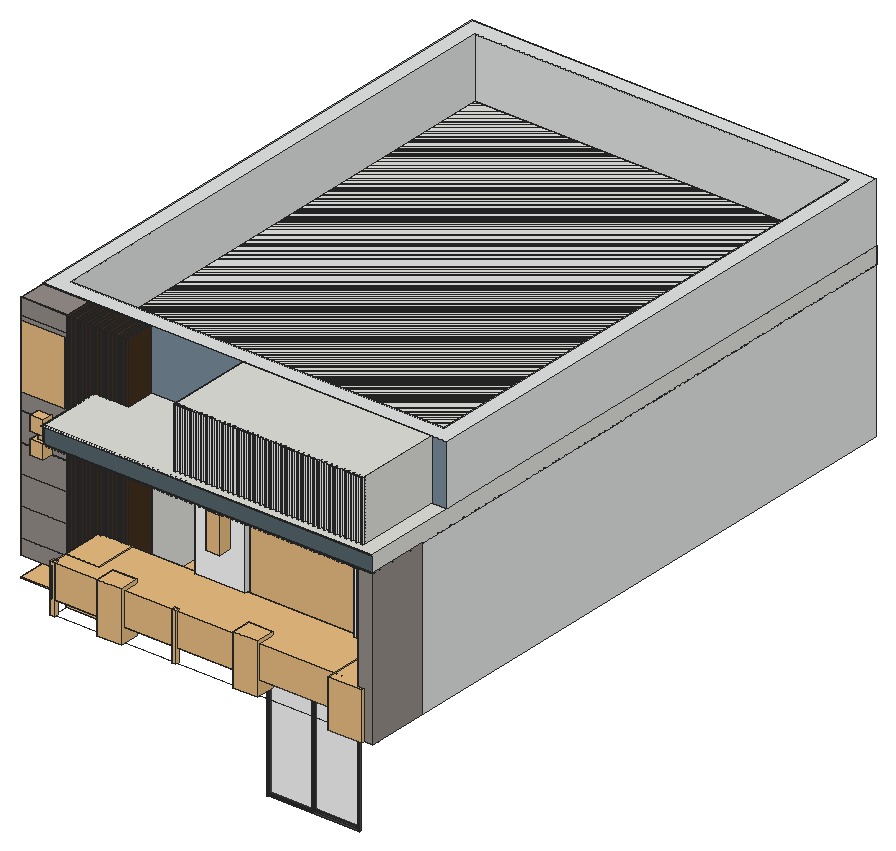
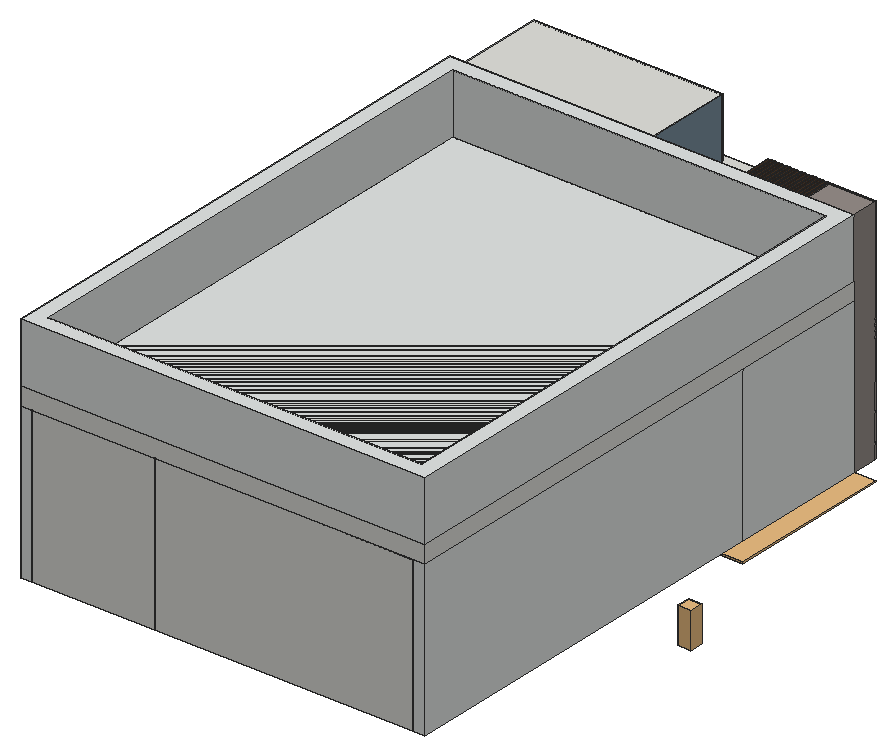
# SketchUp Ruby script. Lengths in inches.
U = 1.inch
M = Sketchup.active_model
def pt(a) = Geom::Point3d.new(a.map { |v| v * U })
def face(e, loops, mat)
  f = e.add_face(loops[0].map { |a| pt(a) })
  loops[1..].each { |l| e.add_face(l.map { |a| pt(a) }).erase! }
  f.material = f.back_material = mat if mat
  f
end
# faces: each face lists its corners as indices into pts; further lists are holes
def faces(e, pts, list, mat = nil) = list.each { |f| face(e, (f[0].is_a?(Array) ? f : [f]).map { |l| l.map { |i| pts[i] } }, mat) }
# xy, xz, yz: faces in a plane at the given z, y or x. An outline is a flat list of corners, or four numbers for a rectangle; further outlines are holes
def ring(l) = l.size == 4 ? [[l[0], l[1]], [l[2], l[1]], [l[2], l[3]], [l[0], l[3]]] : l.each_slice(2).to_a
def flat(e, list, mat, &to3) = list.each { |f| face(e, (f[0].is_a?(Array) ? f : [f]).map { |l| ring(l).map { |u, v| to3.(u, v) } }, mat) }
def xy(e, z, list, mat = nil) = flat(e, list, mat) { |x, y| [x, y, z] }
def xz(e, y, list, mat = nil) = flat(e, list, mat) { |x, z| [x, y, z] }
def yz(e, x, list, mat = nil) = flat(e, list, mat) { |y, z| [x, y, z] }
def lines(e, pts, list) = list.each { |a, b| e.add_line(pt(pts[a]), pt(pts[b])) }
# prism: a flat outline (further loops are holes) pulled along v
def prism(e, loops, v, mat = nil)
  f = face(e, loops, mat); d = Geom::Vector3d.new(v.map { |x| x * U })
  f.pushpull(f.normal.samedirection?(d) ? d.length : -d.length)
end
def box(e, o, s, mat = nil) = prism(e, [[o, [o[0] + s[0], o[1], o[2]], [o[0] + s[0], o[1] + s[1], o[2]], [o[0], o[1] + s[1], o[2]]]], [0, 0, s[2]], mat)
def at(x, y, z, deg = 0) = Geom::Transformation.translation(pt([x, y, z])) * Geom::Transformation.rotation(ORIGIN, Z_AXIS, deg.degrees)
def axes(o, x, y, z) = Geom::Transformation.new([*x, 0, *y, 0, *z, 0, *pt(o).to_a, 1])
def part(name) = M.definitions.add(name)
# library, detail: a bought-in or finely detailed component or shape, given as its bounding box
def library(name, o, s) = part(name).tap { |d| box(d.entities, o, s) }
def detail(e, o, s) = box(e.add_group.entities, o, s)
def put(e, d, t, mat = nil) = e.add_instance(d, t).tap { |i| i.material = mat if mat }
def group(e, t, mat = nil) = e.add_group.tap { |g| g.transformation = t; g.material = mat if mat }.entities
root = M.entities
M.materials.add("Kamosho - kamn7918 33.43cm").color = [255, 255, 255]
M.materials.add("Marble C 150cm").color = [150, 142, 138]
M.materials.add("Plain White Flat 3698829 28cm").color = [227, 230, 229]
M.materials.add("Wall Paint Bumpy 01 Blue 100cm").color = [86, 103, 109]
M.materials.add("Wall Paint Dusk Blue Satin 300cm").color = [122, 143, 157]
M.materials.add("Wood 011 26.84cm").color = [255, 255, 255]
M.materials.add("Wood Amboyan 13.2cm").color = [255, 255, 255]
M.materials.add("Wood Tiles Dark Shiny 03 100cm").color = [68, 48, 33]
M.materials.add("[0135_DarkGray]").color = [81, 81, 81]
M.materials.add("[Translucent Glass Gray]").color = [128, 128, 128]
M.materials["[Translucent Glass Gray]"].alpha = 0.1
c1 = part("PENTEK_RP Fineline 50S_Sliding_DoorCase_E1")
box(c1.entities,[0,0,0],[1.51,3.66,99.27],"[0135_DarkGray]")
c2 = part("PENTEK_RP Fineline 50S_SlidingDooe_Case_E2")
box(c2.entities,[0,0,0],[96.25,3.66,1.51],"[0135_DarkGray]")
c3 = part("pentek_RP Fineline 50S_SlidingDoor_Case")
put(c3.entities,c1,at(97.76,0,0))
put(c3.entities,c2,at(1.51,0,0))
put(c3.entities,c1,at(0,0,0))
put(c3.entities,c2,at(1.51,0,97.76))
c4 = part("PENTEK_RP Fineline 50S_SlidingDoor_GlazingBead_2")
box(c4.entities,[0,0,0],[0.56,0.59,94.39],"[0135_DarkGray]")
c5 = part("PENTEK_RP Fineline 50S_SlidingDoor_Glass")
box(c5.entities,[0,0,0],[46.58,0.16,94.39],"[Translucent Glass Gray]")
c6 = part("PENTEK_RP Fineline 50S_SlidingDoor_GlazingBead")
box(c6.entities,[0,0,0],[45.47,0.59,0.56],"[0135_DarkGray]")
c7 = part("PENTEK_RP Fineline 50S_SlidingDoor_Leaf_E1")
xy(c7.entities,0,[[0,0,0.93,1.97],[0.93,1.57,1.49,1.97]],"[0135_DarkGray]")
xy(c7.entities,96.25,[[0,0,0.93,0,0.93,1.57,1.49,1.57,1.49,1.97,0,1.97]],"[0135_DarkGray]")
xz(c7.entities,0,[[0,0,0.93,96.25]],"[0135_DarkGray]")
xz(c7.entities,1.57,[[0.93,0,1.49,95.32],[0.93,95.32,1.49,96.25]],"[0135_DarkGray]")
xz(c7.entities,1.97,[[0,0,1.49,96.25]],"[0135_DarkGray]")
yz(c7.entities,0,[[0,0,1.97,96.25]],"[0135_DarkGray]")
yz(c7.entities,0.93,[[0,0,1.57,0.93],[0,0.93,1.57,95.32],[0,95.32,1.57,96.25]],"[0135_DarkGray]")
yz(c7.entities,1.49,[[1.57,0,1.97,95.32],[1.57,95.32,1.97,96.25]],"[0135_DarkGray]")
c8 = part("PENTEK_RP Fineline 50S_SlidingDoor_Leaf_E2")
xy(c8.entities,0,[[0,0,0,1.57,0.56,1.57,0.56,1.97,46.02,1.97,46.02,1.57,46.58,1.57,46.58,0]],"[0135_DarkGray]")
xy(c8.entities,0.93,[[0,0,46.58,1.57]],"[0135_DarkGray]")
xy(c8.entities,1.49,[[0.56,1.57,46.02,1.97]],"[0135_DarkGray]")
xz(c8.entities,0,[[0,0,46.58,0.93]],"[0135_DarkGray]")
xz(c8.entities,1.57,[[0,0,0.56,0.93],[46.02,0,46.58,0.93],[0.56,0.93,46.02,1.49]],"[0135_DarkGray]")
xz(c8.entities,1.97,[[0.56,0,46.02,1.49]],"[0135_DarkGray]")
yz(c8.entities,0,[[0,0,1.57,0.93]],"[0135_DarkGray]")
yz(c8.entities,0.56,[[1.57,0,1.97,0.93],[1.57,0.93,1.97,1.49]],"[0135_DarkGray]")
yz(c8.entities,46.02,[[1.57,0,1.97,0.93],[1.57,0.93,1.97,1.49]],"[0135_DarkGray]")
yz(c8.entities,46.58,[[0,0,1.57,0.93]],"[0135_DarkGray]")
c9 = part("PENTEK_RP Fineline S_SlidingDoor_Leaf1")
put(c9.entities,c4,at(0.93,0,0.93))
put(c9.entities,c4,at(46.96,0,0.93))
put(c9.entities,c5,at(1.49,1.42,0.93))
put(c9.entities,c6,at(1.49,0,0.93))
put(c9.entities,c5,at(1.49,0.59,0.93))
put(c9.entities,c7,at(0,0,0))
put(c9.entities,c7,axes([48.44,0,0],[-1,0,0],[0,1,0],[0,0,1]))
put(c9.entities,c8,axes([0.93,0,96.25],[1,0,0],[0,1,0],[0,0,-1]))
put(c9.entities,c8,at(0.93,0,0))
put(c9.entities,c6,at(1.49,0,94.77))
c10 = part("PENTEK_RP Fineline 50S_SlidingDoor_Leaf2")
put(c10.entities,c5,at(1.49,1.42,0.93))
put(c10.entities,c6,at(1.49,0,94.77))
put(c10.entities,c4,at(46.96,0,0.93))
put(c10.entities,c5,at(1.49,0.59,0.93))
put(c10.entities,c4,at(0.93,0,0.93))
put(c10.entities,c7,at(0,0,0))
put(c10.entities,c7,axes([48.44,0,0],[-1,0,0],[0,1,0],[0,0,1]))
put(c10.entities,c6,at(1.49,0,0.93))
put(c10.entities,c8,axes([0.93,0,96.25],[1,0,0],[0,1,0],[0,0,-1]))
put(c10.entities,c8,at(0.93,0,0))
c11 = library("Group\#41",[0,0,0],[10.21,10.21,27.95])
c12 = library("Tlon Light 1950 Ceiling 152 010",[-38.39,-38.39,-3.78],[76.78,76.78,3.41])
c13 = library("Group\#39",[0,0,0],[138,129.875,1])
c14 = library("Potted Plant 13",[-10,-7.28,0],[18.93,15.17,39.22])
c15 = library("Door 243 065",[-19.36,-2.49,0],[38.72,4.98,81.96])
c16 = library("Potted Plant 08",[-13.67,-16.93,0],[26.14,33.37,37.04])
c17 = part("Group\#8")
box(c17.entities,[0,0,0],[96,4.5,120])
c18 = part("Group\#4")
box(c18.entities,[0,0,0],[201,9,120])
c19 = part("Group\#7")
prism(c19.entities,[[[6,4.5,0],[0,4.5,0],[0,4.5,120],[96,4.5,120],[96,4.5,0],[36,4.5,0],[36,4.5,84],[6,4.5,84]]],[0,-4.5,0])
c20 = part("Group\#9")
box(c20.entities,[0,0,0],[96,4.5,120])
c21 = part("Group\#6")
xy(c21.entities,0,[[0,0,90,4.5],[126,0,126,4.5,132,4.5,132,148.5,136.5,148.5,136.5,64.5,160.5,64.5,160.5,60,136.5,60,136.5,0],[190.5,60,190.5,64.5,196.5,64.5,196.5,148.5,201,148.5,201,60]])
xy(c21.entities,84,[[90,0,126,4.5],[160.5,60,190.5,64.5]])
xy(c21.entities,120,[[0,0,136.5,0,136.5,60,201,60,201,148.5,196.5,148.5,196.5,64.5,136.5,64.5,136.5,148.5,132,148.5,132,4.5,0,4.5]])
xz(c21.entities,0,[[0,0,90,0,90,84,126,84,126,0,136.5,0,136.5,120,0,120]])
xz(c21.entities,4.5,[[0,0,0,120,132,120,132,0,126,0,126,84,90,84,90,0]])
xz(c21.entities,60,[[136.5,0,160.5,0,160.5,84,190.5,84,190.5,0,201,0,201,120,136.5,120]])
xz(c21.entities,64.5,[[136.5,0,136.5,120,196.5,120,196.5,0,190.5,0,190.5,84,160.5,84,160.5,0]])
xz(c21.entities,148.5,[[132,0,136.5,120],[196.5,0,201,120]])
yz(c21.entities,0,[[0,0,4.5,120]])
yz(c21.entities,90,[[0,0,4.5,84]])
yz(c21.entities,126,[[0,0,4.5,84]])
yz(c21.entities,132,[[4.5,0,148.5,120]])
yz(c21.entities,136.5,[[0,0,60,120],[64.5,0,148.5,120]])
yz(c21.entities,160.5,[[60,0,64.5,84]])
yz(c21.entities,190.5,[[60,0,64.5,84]])
yz(c21.entities,196.5,[[64.5,0,148.5,120]])
yz(c21.entities,201,[[60,0,148.5,120]])
c22 = part("Vertical panel")
xy(c22.entities,0,[[0,-14.875,2.125,7]])
xy(c22.entities,180,[[0,-14.875,2.125,7]],"Wood Tiles Dark Shiny 03 100cm")
xz(c22.entities,-14.875,[[0,0,2.125,180]],"Wood Tiles Dark Shiny 03 100cm")
xz(c22.entities,7,[[0,0,2.125,180]])
yz(c22.entities,0,[[-14.875,0,7,180]],"Wood Tiles Dark Shiny 03 100cm")
yz(c22.entities,2.125,[[-14.875,0,7,180]],"Wood Tiles Dark Shiny 03 100cm")
c23 = library("Ploe",[1045.01,-6.26,132],[3.15,3.15,37.57])
c24 = part("Group74\#1")
put(c24.entities,c23,at(0,0,0))
put(c24.entities,c23,at(-82.72,0,0))
put(c24.entities,c23,at(-145.86,0,0))
put(c24.entities,c23,at(-240.58,0,0))
put(c24.entities,c23,at(-240.58,45.25,0))
c25 = library("Group75\#1",[805.22,-5.47,143.61],[241.37,46.03,25.18])
c26 = library("DOOR 1",[0,0,0],[82.68,3.9375,84.65])
c27 = library("Spot Light",[-5.1,-5.1,-11.05],[10.2,10.2,11.05])
c28 = library("Lamp Wall Outdoor 94-02",[-1.89,-4.65,-3.17],[3.78,4.65,6.35])
c29 = library("Group\#46",[0,0,0],[39.25,57.0625,1])
c30 = part("Railing baluster")
box(c30.entities,[0,-1,0],[1.1875,1,46.5625],"Wood 011 26.84cm")
xz(root,519.27,[[726.46,251,726.46,252,778.5,252,778.5,251.71,778.26,251.71,778.26,251,776.76,251,776.76,251.71,774.66,251.71,774.66,251,773.16,251,773.16,251.71,771.07,251.71,771.07,251,769.57,251,769.57,251.71,767.48,251.71,767.48,251,765.98,251,765.98,251.78,763.89,251.78,763.89,251,762.39,251,762.39,251.78,760.3,251.78,760.3,251,758.8,251,758.8,251.78,756.7,251.78,756.7,251,755.2,251,755.2,251.78,753.11,251.78,753.11,251,751.61,251,751.61,251.78,749.52,251.78,749.52,251,748.02,251,748.02,251.84,745.93,251.84,745.93,251,744.43,251,744.43,251.84,742.33,251.84,742.33,251,740.83,251,740.83,251.84,738.74,251.84,738.74,251,737.24,251,737.24,251.9,735.15,251.9,735.15,251,733.65,251,733.65,251.9,731.56,251.9,731.56,251,730.06,251,730.06,251.9,727.96,251.9,727.96,251]])
p = [[702.93,344.15,132],[702.93,389.4,132],[766.07,344.15,132],[829.21,344.15,132],[892.36,344.15,132],[955.5,344.15,132],
  [937,374.15,251],[937,354.02,251],[675.04,389.4,296.28],[675.04,389.4,246.07]]
lines(root,p,[[0,1],[0,2],[2,3],[3,4],[4,5],[6,7],[8,9]])
g1 = group(root,at(831,391.58,30))
put(g1,c3,axes([0,0.19,0],[0.72528,0,0],[0,0.49,0],[0,0,0.87512]))
put(g1,c9,axes([1.09,0,1.32],[0.72528,0,0],[0,0.49,0],[0,0,0.87512]))
put(g1,c10,axes([35.77,0.96,1.32],[0.72528,0,0],[0,0.49,0],[0,0,0.87512]))
put(root,c11,at(679.38,511.15,42.52))
put(root,c12,axes([680.94,422.85,115.7],[0.1475,0,0],[0,0.1475,0],[0,0,0.1475]))
put(root,c12,axes([680.94,477.57,115.7],[0.1475,0,0],[0,0.1475,0],[0,0,0.1475]))
put(root,c12,axes([756.5,477.34,115.75],[0.1475,0,0],[0,0.1475,0],[0,0,0.1475]))
put(root,c12,axes([753.27,421.48,115.93],[0.1475,0,0],[0,0.1475,0],[0,0,0.1475]))
put(root,c13,at(640.5,389.4,115.875),"Wood Amboyan 13.2cm")
put(root,c14,at(854.5,349.05,132))
put(root,c14,at(749.45,347.88,132))
put(root,c15,axes([754.52,524.28,132],[0.92977,0,0],[0,-0.44,0],[0,0,1.02]))
put(root,c16,at(715.56,373.65,132))
put(root,c16,at(936.14,353.56,132))
g2 = group(root,at(640.5,339.27,132))
put(g2,c17,at(210,486,0))
put(g2,c18,at(9,481.5,0))
g3 = group(g2,at(306,0,0))
box(g3,[0,48,0],[9,442.5,120],"Plain White Flat 3698829 28cm")
put(g2,c19,at(210,433.5,0))
g4 = group(g2,at(0,0,0))
box(g4,[0,180,0],[9,310.5,120],"Plain White Flat 3698829 28cm")
put(g2,c20,at(210,225,0))
g5 = group(g2,at(9,48,0))
xy(g5,0,[[129,0,129,132,123,132,123,141,138,141,138,9,297,9,297,0],[0,132,87,141]])
xy(g5,6,[[167.625,0,253.5,9]])
xy(g5,84,[[87,132,123,141]])
xy(g5,112.4375,[[167.625,0,253.5,9]])
xy(g5,120,[[129,0,297,0,297,9,138,9,138,141,0,141,0,132,129,132]])
xz(g5,0,[[[129,0,297,120],[167.625,6,253.5,112.4375]]],"Kamosho - kamn7918 33.43cm")
xz(g5,9,[[[138,0,297,120],[167.625,6,253.5,112.4375]]])
xz(g5,132,[[0,0,87,0,87,84,123,84,123,0,129,0,129,120,0,120]],"Kamosho - kamn7918 33.43cm")
xz(g5,141,[[0,0,0,120,138,120,138,0,123,0,123,84,87,84,87,0]])
yz(g5,0,[[132,0,141,120]])
yz(g5,87,[[132,0,141,84]])
yz(g5,123,[[132,0,141,84]])
yz(g5,129,[[0,0,132,120]],"Kamosho - kamn7918 33.43cm")
yz(g5,138,[[9,0,141,120]])
yz(g5,167.625,[[0,6,9,112.4375]])
yz(g5,253.5,[[0,6,9,112.4375]])
yz(g5,297,[[0,0,9,120]])
put(g2,c21,at(9,333,0))
g6 = group(root,at(640.5,404.27,132))
box(g6,[0,-13.875,0],[35.9375,20.875,180],"Marble C 150cm")
g7 = group(root,at(640.5,389.4,132),"Marble C 150cm")
box(g7,[34.54,0,123.52],[1.4,1,21.92],"Marble C 150cm")
xy(g7,0,[[0,0,35.9375,1]],"Marble C 150cm")
xy(g7,12,[[0,0,35.9375,1]],"Marble C 150cm")
xy(g7,12.31,[[0,0,35.9375,1]],"Marble C 150cm")
xy(g7,34.24,[[0,0,35.9375,1]],"Marble C 150cm")
xy(g7,34.56,[[0,0,35.9375,1]],"Marble C 150cm")
xy(g7,56.48,[[0,0,35.9375,1]],"Marble C 150cm")
xy(g7,56.8,[[0,0,35.9375,1]],"Marble C 150cm")
xy(g7,78.72,[[0,0,35.9375,1]],"Marble C 150cm")
xy(g7,79.04,[[0,0,35.9375,1]],"Marble C 150cm")
xy(g7,100.96,[[0,0,35.9375,1]],"Marble C 150cm")
xy(g7,101.28,[[0,0,35.9375,1]],"Marble C 150cm")
xy(g7,114.07,[[0,0,34.54,1]],"Marble C 150cm")
xy(g7,123.2,[[34.54,0,35.9375,1]],"Marble C 150cm")
xy(g7,145.76,[[34.54,0,35.9375,1]],"Marble C 150cm")
xy(g7,164.28,[[0,0,34.54,1]],"Marble C 150cm")
xy(g7,167.69,[[0,0,35.9375,1]],"Marble C 150cm")
xy(g7,168,[[0,0,35.9375,1]],"Marble C 150cm")
xy(g7,180,[[0,0,35.9375,1]],"Marble C 150cm")
xz(g7,0,[[0,0,35.9375,12],[0,12.31,35.9375,34.24],[0,34.56,35.9375,56.48],[0,56.8,35.9375,78.72],[0,79.04,35.9375,100.96],
  [0,101.28,35.9375,101.28,35.9375,123.2,34.54,123.2,34.54,114.07,0,114.07],[34.54,145.76,35.9375,145.76,35.9375,167.69,0,167.69,0,164.28,34.54,164.28],[0,168,35.9375,180]],"Marble C 150cm")
xz(g7,1,[[0,0,35.9375,12],[0,12,35.9375,12.31],[0,12.31,35.9375,34.24],[0,34.24,35.9375,34.56],[0,34.56,35.9375,56.48],
  [0,56.48,35.9375,56.8],[0,56.8,35.9375,78.72],[0,78.72,35.9375,79.04],[0,79.04,35.9375,100.96],[0,100.96,35.9375,101.28],
  [0,101.28,0,114.07,34.54,114.07,34.54,123.2,35.9375,123.2,35.9375,101.28],[34.54,145.76,34.54,164.28,0,164.28,0,167.69,35.9375,167.69,35.9375,145.76],[0,167.69,35.9375,168],[0,168,35.9375,180]],"Marble C 150cm")
yz(g7,0,[[0,0,1,12],[0,12.31,1,34.24],[0,34.56,1,56.48],[0,56.8,1,78.72],[0,79.04,1,100.96],
  [0,101.28,1,114.07],[0,164.28,1,167.69],[0,168,1,180]],"Marble C 150cm")
yz(g7,34.54,[[0,114.07,1,123.2],[0,145.76,1,164.28]],"Marble C 150cm")
yz(g7,35.9375,[[0,0,1,12],[0,12.31,1,34.24],[0,34.56,1,56.48],[0,56.8,1,78.72],[0,79.04,1,100.96],
  [0,101.28,1,123.2],[0,145.76,1,167.69],[0,168,1,180]],"Marble C 150cm")
p = [[35.9375,1,123.52],[35.9375,1,123.2],[35.9375,1,145.76],[35.9375,1,145.44],[34.54,0,123.52],[34.54,0,123.2],
  [34.54,0,145.76],[34.54,0,145.44]]
lines(g7,p,[[0,1],[2,3],[4,5],[6,7]])
g8 = group(root,at(676.44,389.4,132))
put(g8,c22,at(46.49,14.875,0))
put(g8,c22,at(34.69,14.875,0))
put(g8,c22,at(31.8,14.875,0))
put(g8,c22,at(37.58,14.875,0))
put(g8,c22,at(43.36,14.875,0))
put(g8,c22,at(0,14.875,0),"Wood Tiles Dark Shiny 03 100cm")
put(g8,c22,at(23.13,14.875,0))
put(g8,c22,at(20.24,14.875,0))
put(g8,c22,at(40.47,14.875,0))
put(g8,c22,at(17.35,14.875,0))
put(g8,c22,at(28.91,14.875,0))
put(g8,c22,at(26.02,14.875,0))
put(g8,c22,at(8.67,14.875,0))
put(g8,c22,at(2.89,14.875,0),"Wood Tiles Dark Shiny 03 100cm")
put(g8,c22,at(5.78,14.875,0))
put(g8,c22,at(11.5625,14.875,0))
put(g8,c22,at(14.45,14.875,0))
g9 = group(root,at(943.5,339.27,132),"Marble C 150cm")
prism(g9,[[[0,0,0],[12,0,0],[12,0,120],[0,0,120],[0,0,119]]],[0,48,0])
g10 = group(root,at(640.5,411.27,132))
xy(g10,120,[[0,0,85.93,0,85.93,108,81.43,108,81.43,9,9,9,9,108,0,108]])
xz(g10,0,[[0,0,85.93,120]])
xz(g10,9,[[9,0,81.43,120]])
xz(g10,108,[[0,0,9,120],[81.43,0,85.93,120]])
yz(g10,0,[[0,0,108,120]],"Plain White Flat 3698829 28cm")
yz(g10,9,[[9,0,108,120]])
yz(g10,81.43,[[9,0,108,120]])
yz(g10,85.93,[[0,0,108,120]])
g11 = group(root,at(701.35,342.57,132))
put(g11,c24,at(-804.4375,6.26,-132))
put(g11,c25,at(-804.4375,6.26,-132))
g12 = group(root,at(903,386.27,132),"Wood 011 26.84cm")
prism(g12,[[[0,1,0],[40.5,1,0],[40.5,0,0],[38.5,0,0],[38.5,0.5,0],[36.65,0.5,0],[36.65,0,0],[34.65,0,0],[34.65,0.5,0],[32.8,0.5,0],[32.8,0,0],[30.8,0,0],[30.8,0.5,0],[28.95,0.5,0],[28.95,0,0],[26.95,0,0],[26.95,0.5,0],[25.1,0.5,0],[25.1,0,0],[23.1,0,0],[23.1,0.5,0],[21.25,0.5,0],[21.25,0,0],[19.25,0,0],[19.25,0.5,0],[17.4,0.5,0],[17.4,0,0],[15.4,0,0],[15.4,0.5,0],[13.55,0.5,0],[13.55,0,0],[11.55,0,0],[11.55,0.5,0],[9.7,0.5,0],[9.7,0,0],[7.7,0,0],[7.7,0.5,0],[5.85,0.5,0],[5.85,0,0],[3.85,0,0],[3.85,0.5,0],[2,0.5,0],[2,0,0],[0,0,0]]],[0,0,119])
put(root,c26,axes([817.13,391.77,138],[1.03868,0,0],[0,1,0],[0,0,1.25745]))
put(root,c11,at(795.32,377.07,195.11))
put(root,c27,at(659.61,386.45,221.45))
put(root,c28,at(659.79,389.37,224.6))
put(root,c27,axes([659.61,386.45,227.29],[1,0,0],[0,1,0],[0,0,-1]))
put(root,c29,axes([640.5,390.4,246.07],[0.88,0,0],[0,0,0.88],[0,-0.88,0]),"Marble C 150cm")
put(root,c12,axes([752.5,418.16,250.7],[0.1475,0,0],[0,0.1475,0],[0,0,0.1475]))
put(root,c12,axes([873.18,360.65,250.77],[0.1475,0,0],[0,0.1475,0],[0,0,0.1475]))
put(root,c12,axes([801.06,360.65,250.77],[0.1475,0,0],[0,0.1475,0],[0,0,0.1475]))
put(root,c12,axes([718.04,360.65,250.77],[0.1475,0,0],[0,0.1475,0],[0,0,0.1475]))
put(root,c12,axes([925.98,360.65,250.77],[0.1475,0,0],[0,0.1475,0],[0,0,0.1475]))
g13 = group(root,at(698.8,339.27,251),"Wood Amboyan 13.2cm")
g14 = group(g13,at(27.66,0,0))
xy(g14,0,[[0,0,1.5,180],[3.59,0,5.09,180],[7.18,0,8.68,180],[10.78,0,12.28,180],[14.37,0,15.87,180],
  [17.96,0,19.46,180],[21.55,0,23.05,180],[25.15,0,26.65,180],[28.74,0,30.24,180],[32.33,0,33.83,180],
  [35.92,0,37.42,180],[39.52,0,41.02,180],[43.11,0,44.61,180],[46.7,0,48.2,180],[50.29,0,51.79,180],
  [53.88,0,55.38,48],[57.48,0,58.98,48],[61.07,0,62.57,48],[64.66,0,66.16,48],[68.25,0,69.75,48],
  [71.85,0,73.35,48],[75.4375,0,76.9375,48],[79.03,0,80.53,48],[82.62,0,84.12,48],[86.21,0,87.71,48],
  [89.81,0,91.31,48],[93.4,0,94.9,48],[96.99,0,98.49,48],[100.58,0,102.08,48],[104.18,0,105.68,48],
  [107.77,0,109.27,48],[111.36,0,112.86,48],[114.95,0,116.45,48],[118.55,0,120.05,48],[122.14,0,123.64,48],
  [125.73,0,127.23,48],[129.32,0,130.82,48],[132.91,0,134.41,48],[136.51,0,138.01,48],[140.1,0,141.6,48],
  [143.69,0,145.19,48],[147.28,0,148.78,48],[150.875,0,152.375,48],[154.47,0,155.97,48],[158.0625,0,159.5625,48],
  [161.65,0,163.15,48],[165.25,0,166.75,48],[168.84,0,170.34,48],[172.43,0,173.93,48],[176.02,0,177.52,48],
  [179.61,0,181.11,48],[183.21,0,184.71,48],[186.8,0,188.3,48],[190.39,0,191.89,48],[193.98,0,195.48,48],
  [197.58,0,199.08,48],[201.17,0,202.67,48],[204.76,0,206.26,48],[208.35,0,209.85,48],[211.94,0,213.44,48],
  [215.54,0,217.04,48]])
xy(g14,0.59,[[102.08,0,104.18,48],[105.68,0,107.77,48],[109.27,0,111.36,48],[112.86,0,114.95,48],[116.45,0,118.55,48],
  [120.05,0,122.14,48],[123.64,0,125.73,48],[127.23,0,129.32,48],[130.82,0,132.91,48],[134.41,0,136.51,48],
  [138.01,0,140.1,48],[141.6,0,143.69,48],[145.19,0,147.28,48],[148.78,0,150.875,48],[152.375,0,154.47,48],
  [155.97,0,158.0625,48],[159.5625,0,161.65,48]])
xy(g14,0.71,[[41.02,0,43.11,180],[44.61,0,46.7,180],[48.2,0,50.29,180],[51.79,0,51.79,180,52.04,180,52.04,48,53.88,48,53.88,0],[55.38,0,57.48,48],
  [58.98,0,61.07,48],[62.57,0,64.66,48],[66.16,0,68.25,48],[69.75,0,71.85,48],[73.35,0,75.4375,48],
  [76.9375,0,79.03,48],[80.53,0,82.62,48],[84.12,0,86.21,48],[87.71,0,89.81,48],[91.31,0,93.4,48],
  [94.9,0,96.99,48],[98.49,0,100.58,48]])
xy(g14,0.78,[[23.05,0,25.15,180],[26.65,0,28.74,180],[30.24,0,32.33,180],[33.83,0,35.92,180],[37.42,0,39.52,180]])
xy(g14,0.84,[[12.28,0,14.37,180],[15.87,0,17.96,180],[19.46,0,21.55,180]])
xy(g14,0.86,[[163.15,0,165.25,48],[166.75,0,168.84,48]])
xy(g14,0.9,[[1.5,0,3.59,180],[5.09,0,7.18,180],[8.68,0,10.78,180],[170.34,0,172.43,48],[173.93,0,176.02,48],
  [177.52,0,179.61,48],[181.11,0,183.21,48],[184.71,0,186.8,48],[188.3,0,190.39,48],[191.89,0,193.98,48],
  [195.48,0,197.58,48],[199.08,0,201.17,48],[202.67,0,204.76,48],[206.26,0,208.35,48],[209.85,0,211.94,48],
  [213.44,0,215.54,48]])
xy(g14,1,[[0,0,217.04,0,217.04,48,52.04,48,52.04,180,0,180]])
xz(g14,0,[[0,0,1.5,0,1.5,0.9,3.59,0.9,3.59,0,5.09,0,5.09,0.9,7.18,0.9,7.18,0,8.68,0,8.68,0.9,10.78,0.9,10.78,0,12.28,0,12.28,0.84,14.37,0.84,14.37,0,15.87,0,15.87,0.84,17.96,0.84,17.96,0,19.46,0,19.46,0.84,21.55,0.84,21.55,0,23.05,0,23.05,0.78,25.15,0.78,25.15,0,26.65,0,26.65,0.78,28.74,0.78,28.74,0,30.24,0,30.24,0.78,32.33,0.78,32.33,0,33.83,0,33.83,0.78,35.92,0.78,35.92,0,37.42,0,37.42,0.78,39.52,0.78,39.52,0,41.02,0,41.02,0.71,43.11,0.71,43.11,0,44.61,0,44.61,0.71,46.7,0.71,46.7,0,48.2,0,48.2,0.71,50.29,0.71,50.29,0,51.79,0,51.79,0.71,53.88,0.71,53.88,0,55.38,0,55.38,0.71,57.48,0.71,57.48,0,58.98,0,58.98,0.71,61.07,0.71,61.07,0,62.57,0,62.57,0.71,64.66,0.71,64.66,0,66.16,0,66.16,0.71,68.25,0.71,68.25,0,69.75,0,69.75,0.71,71.85,0.71,71.85,0,73.35,0,73.35,0.71,75.4375,0.71,75.4375,0,76.9375,0,76.9375,0.71,79.03,0.71,79.03,0,80.53,0,80.53,0.71,82.62,0.71,82.62,0,84.12,0,84.12,0.71,86.21,0.71,86.21,0,87.71,0,87.71,0.71,89.81,0.71,89.81,0,91.31,0,91.31,0.71,93.4,0.71,93.4,0,94.9,0,94.9,0.71,96.99,0.71,96.99,0,98.49,0,98.49,0.71,100.58,0.71,100.58,0,102.08,0,102.08,0.59,104.18,0.59,104.18,0,105.68,0,105.68,0.59,107.77,0.59,107.77,0,109.27,0,109.27,0.59,111.36,0.59,111.36,0,112.86,0,112.86,0.59,114.95,0.59,114.95,0,116.45,0,116.45,0.59,118.55,0.59,118.55,0,120.05,0,120.05,0.59,122.14,0.59,122.14,0,123.64,0,123.64,0.59,125.73,0.59,125.73,0,127.23,0,127.23,0.59,129.32,0.59,129.32,0,130.82,0,130.82,0.59,132.91,0.59,132.91,0,134.41,0,134.41,0.59,136.51,0.59,136.51,0,138.01,0,138.01,0.59,140.1,0.59,140.1,0,141.6,0,141.6,0.59,143.69,0.59,143.69,0,145.19,0,145.19,0.59,147.28,0.59,147.28,0,148.78,0,148.78,0.59,150.875,0.59,150.875,0,152.375,0,152.375,0.59,154.47,0.59,154.47,0,155.97,0,155.97,0.59,158.0625,0.59,158.0625,0,159.5625,0,159.5625,0.59,161.65,0.59,161.65,0,163.15,0,163.15,0.86,165.25,0.86,165.25,0,166.75,0,166.75,0.86,168.84,0.86,168.84,0,170.34,0,170.34,0.9,172.43,0.9,172.43,0,173.93,0,173.93,0.9,176.02,0.9,176.02,0,177.52,0,177.52,0.9,179.61,0.9,179.61,0,181.11,0,181.11,0.9,183.21,0.9,183.21,0,184.71,0,184.71,0.9,186.8,0.9,186.8,0,188.3,0,188.3,0.9,190.39,0.9,190.39,0,191.89,0,191.89,0.9,193.98,0.9,193.98,0,195.48,0,195.48,0.9,197.58,0.9,197.58,0,199.08,0,199.08,0.9,201.17,0.9,201.17,0,202.67,0,202.67,0.9,204.76,0.9,204.76,0,206.26,0,206.26,0.9,208.35,0.9,208.35,0,209.85,0,209.85,0.9,211.94,0.9,211.94,0,213.44,0,213.44,0.9,215.54,0.9,215.54,0,217.04,0,217.04,1,0,1]])
xz(g14,48,[[53.88,0,53.88,0.71,52.04,0.71,52.04,1,217.04,1,217.04,0,215.54,0,215.54,0.9,213.44,0.9,213.44,0,211.94,0,211.94,0.9,209.85,0.9,209.85,0,208.35,0,208.35,0.9,206.26,0.9,206.26,0,204.76,0,204.76,0.9,202.67,0.9,202.67,0,201.17,0,201.17,0.9,199.08,0.9,199.08,0,197.58,0,197.58,0.9,195.48,0.9,195.48,0,193.98,0,193.98,0.9,191.89,0.9,191.89,0,190.39,0,190.39,0.9,188.3,0.9,188.3,0,186.8,0,186.8,0.9,184.71,0.9,184.71,0,183.21,0,183.21,0.9,181.11,0.9,181.11,0,179.61,0,179.61,0.9,177.52,0.9,177.52,0,176.02,0,176.02,0.9,173.93,0.9,173.93,0,172.43,0,172.43,0.9,170.34,0.9,170.34,0,168.84,0,168.84,0.86,166.75,0.86,166.75,0,165.25,0,165.25,0.86,163.15,0.86,163.15,0,161.65,0,161.65,0.59,159.5625,0.59,159.5625,0,158.0625,0,158.0625,0.59,155.97,0.59,155.97,0,154.47,0,154.47,0.59,152.375,0.59,152.375,0,150.875,0,150.875,0.59,148.78,0.59,148.78,0,147.28,0,147.28,0.59,145.19,0.59,145.19,0,143.69,0,143.69,0.59,141.6,0.59,141.6,0,140.1,0,140.1,0.59,138.01,0.59,138.01,0,136.51,0,136.51,0.59,134.41,0.59,134.41,0,132.91,0,132.91,0.59,130.82,0.59,130.82,0,129.32,0,129.32,0.59,127.23,0.59,127.23,0,125.73,0,125.73,0.59,123.64,0.59,123.64,0,122.14,0,122.14,0.59,120.05,0.59,120.05,0,118.55,0,118.55,0.59,116.45,0.59,116.45,0,114.95,0,114.95,0.59,112.86,0.59,112.86,0,111.36,0,111.36,0.59,109.27,0.59,109.27,0,107.77,0,107.77,0.59,105.68,0.59,105.68,0,104.18,0,104.18,0.59,102.08,0.59,102.08,0,100.58,0,100.58,0.71,98.49,0.71,98.49,0,96.99,0,96.99,0.71,94.9,0.71,94.9,0,93.4,0,93.4,0.71,91.31,0.71,91.31,0,89.81,0,89.81,0.71,87.71,0.71,87.71,0,86.21,0,86.21,0.71,84.12,0.71,84.12,0,82.62,0,82.62,0.71,80.53,0.71,80.53,0,79.03,0,79.03,0.71,76.9375,0.71,76.9375,0,75.4375,0,75.4375,0.71,73.35,0.71,73.35,0,71.85,0,71.85,0.71,69.75,0.71,69.75,0,68.25,0,68.25,0.71,66.16,0.71,66.16,0,64.66,0,64.66,0.71,62.57,0.71,62.57,0,61.07,0,61.07,0.71,58.98,0.71,58.98,0,57.48,0,57.48,0.71,55.38,0.71,55.38,0]])
yz(g14,0,[[0,0,180,1]])
yz(g14,1.5,[[0,0,180,0.9]])
yz(g14,3.59,[[0,0,180,0.9]])
yz(g14,5.09,[[0,0,180,0.9]])
yz(g14,7.18,[[0,0,180,0.9]])
yz(g14,8.68,[[0,0,180,0.9]])
yz(g14,10.78,[[0,0,180,0.9]])
yz(g14,12.28,[[0,0,180,0.84]])
yz(g14,14.37,[[0,0,180,0.84]])
yz(g14,15.87,[[0,0,180,0.84]])
yz(g14,17.96,[[0,0,180,0.84]])
yz(g14,19.46,[[0,0,180,0.84]])
yz(g14,21.55,[[0,0,180,0.84]])
yz(g14,23.05,[[0,0,180,0.78]])
yz(g14,25.15,[[0,0,180,0.78]])
yz(g14,26.65,[[0,0,180,0.78]])
yz(g14,28.74,[[0,0,180,0.78]])
yz(g14,30.24,[[0,0,180,0.78]])
yz(g14,32.33,[[0,0,180,0.78]])
yz(g14,33.83,[[0,0,180,0.78]])
yz(g14,35.92,[[0,0,180,0.78]])
yz(g14,37.42,[[0,0,180,0.78]])
yz(g14,39.52,[[0,0,180,0.78]])
yz(g14,41.02,[[0,0,180,0.71]])
yz(g14,43.11,[[0,0,180,0.71]])
yz(g14,44.61,[[0,0,180,0.71]])
yz(g14,46.7,[[0,0,180,0.71]])
yz(g14,48.2,[[0,0,180,0.71]])
yz(g14,50.29,[[0,0,180,0.71]])
yz(g14,51.79,[[0,0,180,0.71]])
yz(g14,52.04,[[48,0.71,180,1]])
yz(g14,53.88,[[0,0,48,0.71]])
yz(g14,55.38,[[0,0,48,0.71]])
yz(g14,57.48,[[0,0,48,0.71]])
yz(g14,58.98,[[0,0,48,0.71]])
yz(g14,61.07,[[0,0,48,0.71]])
yz(g14,62.57,[[0,0,48,0.71]])
yz(g14,64.66,[[0,0,48,0.71]])
yz(g14,66.16,[[0,0,48,0.71]])
yz(g14,68.25,[[0,0,48,0.71]])
yz(g14,69.75,[[0,0,48,0.71]])
yz(g14,71.85,[[0,0,48,0.71]])
yz(g14,73.35,[[0,0,48,0.71]])
yz(g14,75.4375,[[0,0,48,0.71]])
yz(g14,76.9375,[[0,0,48,0.71]])
yz(g14,79.03,[[0,0,48,0.71]])
yz(g14,80.53,[[0,0,48,0.71]])
yz(g14,82.62,[[0,0,48,0.71]])
yz(g14,84.12,[[0,0,48,0.71]])
yz(g14,86.21,[[0,0,48,0.71]])
yz(g14,87.71,[[0,0,48,0.71]])
yz(g14,89.81,[[0,0,48,0.71]])
yz(g14,91.31,[[0,0,48,0.71]])
yz(g14,93.4,[[0,0,48,0.71]])
yz(g14,94.9,[[0,0,48,0.71]])
yz(g14,96.99,[[0,0,48,0.71]])
yz(g14,98.49,[[0,0,48,0.71]])
yz(g14,100.58,[[0,0,48,0.71]])
yz(g14,102.08,[[0,0,48,0.59]])
yz(g14,104.18,[[0,0,48,0.59]])
yz(g14,105.68,[[0,0,48,0.59]])
yz(g14,107.77,[[0,0,48,0.59]])
yz(g14,109.27,[[0,0,48,0.59]])
yz(g14,111.36,[[0,0,48,0.59]])
yz(g14,112.86,[[0,0,48,0.59]])
yz(g14,114.95,[[0,0,48,0.59]])
yz(g14,116.45,[[0,0,48,0.59]])
yz(g14,118.55,[[0,0,48,0.59]])
yz(g14,120.05,[[0,0,48,0.59]])
yz(g14,122.14,[[0,0,48,0.59]])
yz(g14,123.64,[[0,0,48,0.59]])
yz(g14,125.73,[[0,0,48,0.59]])
yz(g14,127.23,[[0,0,48,0.59]])
yz(g14,129.32,[[0,0,48,0.59]])
yz(g14,130.82,[[0,0,48,0.59]])
yz(g14,132.91,[[0,0,48,0.59]])
yz(g14,134.41,[[0,0,48,0.59]])
yz(g14,136.51,[[0,0,48,0.59]])
yz(g14,138.01,[[0,0,48,0.59]])
yz(g14,140.1,[[0,0,48,0.59]])
yz(g14,141.6,[[0,0,48,0.59]])
yz(g14,143.69,[[0,0,48,0.59]])
yz(g14,145.19,[[0,0,48,0.59]])
yz(g14,147.28,[[0,0,48,0.59]])
yz(g14,148.78,[[0,0,48,0.59]])
yz(g14,150.875,[[0,0,48,0.59]])
yz(g14,152.375,[[0,0,48,0.59]])
yz(g14,154.47,[[0,0,48,0.59]])
yz(g14,155.97,[[0,0,48,0.59]])
yz(g14,158.0625,[[0,0,48,0.59]])
yz(g14,159.5625,[[0,0,48,0.59]])
yz(g14,161.65,[[0,0,48,0.59]])
yz(g14,163.15,[[0,0,48,0.86]])
yz(g14,165.25,[[0,0,48,0.86]])
yz(g14,166.75,[[0,0,48,0.86]])
yz(g14,168.84,[[0,0,48,0.86]])
yz(g14,170.34,[[0,0,48,0.9]])
yz(g14,172.43,[[0,0,48,0.9]])
yz(g14,173.93,[[0,0,48,0.9]])
yz(g14,176.02,[[0,0,48,0.9]])
yz(g14,177.52,[[0,0,48,0.9]])
yz(g14,179.61,[[0,0,48,0.9]])
yz(g14,181.11,[[0,0,48,0.9]])
yz(g14,183.21,[[0,0,48,0.9]])
yz(g14,184.71,[[0,0,48,0.9]])
yz(g14,186.8,[[0,0,48,0.9]])
yz(g14,188.3,[[0,0,48,0.9]])
yz(g14,190.39,[[0,0,48,0.9]])
yz(g14,191.89,[[0,0,48,0.9]])
yz(g14,193.98,[[0,0,48,0.9]])
yz(g14,195.48,[[0,0,48,0.9]])
yz(g14,197.58,[[0,0,48,0.9]])
yz(g14,199.08,[[0,0,48,0.9]])
yz(g14,201.17,[[0,0,48,0.9]])
yz(g14,202.67,[[0,0,48,0.9]])
yz(g14,204.76,[[0,0,48,0.9]])
yz(g14,206.26,[[0,0,48,0.9]])
yz(g14,208.35,[[0,0,48,0.9]])
yz(g14,209.85,[[0,0,48,0.9]])
yz(g14,211.94,[[0,0,48,0.9]])
yz(g14,213.44,[[0,0,48,0.9]])
yz(g14,215.54,[[0,0,48,0.9]])
g15 = group(g13,at(0,0,0))
prism(g15,[[[0,64.99,1],[27.66,64.99,1],[27.66,64.99,0.0625],[25.54,64.99,0.0625],[25.54,64.99,0.9],[24.04,64.99,0.9],[24.04,64.99,0],[23.13,64.99,0],[23.13,64.99,0.9],[21.63,64.99,0.9],[21.63,64.99,0],[20.73,64.99,0],[20.73,64.99,0.9],[19.23,64.99,0.9],[19.23,64.99,0],[18.33,64.99,0],[18.33,64.99,0.9],[16.83,64.99,0.9],[16.83,64.99,0],[15.92,64.99,0],[15.92,64.99,0.9],[14.42,64.99,0.9],[14.42,64.99,0],[13.52,64.99,0],[13.52,64.99,0.9],[12.02,64.99,0.9],[12.02,64.99,0],[11.12,64.99,0],[11.12,64.99,0.9],[9.62,64.99,0.9],[9.62,64.99,0],[8.71,64.99,0],[8.71,64.99,0.9],[7.21,64.99,0.9],[7.21,64.99,0],[6.31,64.99,0],[6.31,64.99,0.9],[4.81,64.99,0.9],[4.81,64.99,0],[3.9,64.99,0],[3.9,64.99,0.9],[2.4,64.99,0.9],[2.4,64.99,0],[1.5,64.99,0],[1.5,64.99,0.9],[0,64.99,0.9]]],[0,-64.99,0])
g16 = group(root,at(640.5,333.91,252))
xy(g16,0,[[57.86,4.93,57.86,70.37,81.43,70.37,81.43,77.37,0,77.37,0,495.87,315,495.87,315,4.93]])
xy(g16,0.375,[[57.86,4.93,315,4.93,315,5.37,58.3,5.37,58.3,70.37,57.86,70.37]])
xy(g16,13.125,[[57.61,3.8,57.61,70.37,58.3,70.37,58.3,5.37,315,5.37,315,3.8]])
xy(g16,13.4375,[[57.61,3.8,315,3.8,315,495.87,0,495.87,0,77.37,81.43,77.37,81.43,70.37,57.61,70.37]])
xz(g16,3.8,[[57.61,13.125,315,13.4375]])
xz(g16,4.93,[[57.86,0,315,0.375]])
xz(g16,5.37,[[58.3,0.375,315,13.125]],"Wall Paint Bumpy 01 Blue 100cm")
xz(g16,70.37,[[57.86,0,57.86,0.375,58.3,0.375,58.3,13.125,57.61,13.125,57.61,13.4375,81.43,13.4375,81.43,0]])
xz(g16,77.37,[[0,0,81.43,13.4375]])
xz(g16,495.87,[[0,0,315,13.4375]])
yz(g16,0,[[77.37,0,495.87,13.4375]])
yz(g16,57.61,[[3.8,13.125,70.37,13.4375]])
yz(g16,57.86,[[4.93,0,70.37,0.375]])
yz(g16,58.3,[[5.37,0.375,70.37,13.125]],"Wall Paint Bumpy 01 Blue 100cm")
yz(g16,81.43,[[70.37,0,77.37,13.4375]])
yz(g16,315,[[4.93,0,495.87,0,495.87,13.4375,3.8,13.4375,3.8,13.125,5.37,13.125,5.37,0.375,4.93,0.375]])
g17 = group(root,at(796.49,345.15,265.4375),"Wood 011 26.84cm")
xy(g17,0,[[0,0,147.01,1]])
xy(g17,46.5625,[[0,0,147.01,1]])
xz(g17,0,[[1.1875,0,147.01,46.5625]])
xz(g17,1,[[0,0,147.01,46.5625]])
yz(g17,0,[[0,0,1,46.5625]])
yz(g17,147.01,[[0,0,1,46.5625]])
put(g17,c30,at(0,0,0))
put(g17,c30,at(145.83,0,0))
put(g17,c30,at(4.17,0,0))
put(g17,c30,at(8.33,0,0))
put(g17,c30,at(12.5,0,0))
put(g17,c30,at(16.67,0,0))
put(g17,c30,at(20.83,0,0))
put(g17,c30,at(25,0,0))
put(g17,c30,at(29.17,0,0))
put(g17,c30,at(33.33,0,0))
put(g17,c30,at(37.5,0,0))
put(g17,c30,at(41.66,0,0))
put(g17,c30,at(45.83,0,0))
put(g17,c30,at(50,0,0))
put(g17,c30,at(54.16,0,0))
put(g17,c30,at(58.33,0,0))
put(g17,c30,at(62.5,0,0))
put(g17,c30,at(66.66,0,0))
put(g17,c30,at(70.83,0,0))
put(g17,c30,at(75,0,0))
put(g17,c30,at(79.16,0,0))
put(g17,c30,at(83.33,0,0))
put(g17,c30,at(87.5,0,0))
put(g17,c30,at(91.66,0,0))
put(g17,c30,at(95.83,0,0))
put(g17,c30,at(100,0,0))
put(g17,c30,at(104.16,0,0))
put(g17,c30,at(108.33,0,0))
put(g17,c30,at(112.49,0,0))
put(g17,c30,at(116.66,0,0))
put(g17,c30,at(120.83,0,0))
put(g17,c30,at(124.99,0,0))
put(g17,c30,at(129.16,0,0))
put(g17,c30,at(133.33,0,0))
put(g17,c30,at(137.49,0,0))
put(g17,c30,at(141.66,0,0))
g18 = group(root,at(796.49,346.15,265.4375))
xy(g18,0,[[0,0,147.01,65.125]])
xy(g18,46.5625,[[0,-2,147.01,0],[0,0,147.01,65.125]])
xy(g18,46.875,[[0,-2,147.01,65.125]])
xz(g18,-2,[[0,46.5625,147.01,46.875]])
xz(g18,0,[[0,0,147.01,46.5625]])
xz(g18,65.125,[[0,0,147.01,46.5625],[0,46.5625,147.01,46.875]])
yz(g18,0,[[-2,46.5625,65.125,46.875]])
yz(g18,0,[[0,0,65.125,46.5625]],"Wall Paint Dusk Blue Satin 300cm")
yz(g18,147.01,[[0,0,65.125,46.5625],[-2,46.5625,65.125,46.875]])
g19 = group(root,at(640.5,411.27,265.4375),"Plain White Flat 3698829 28cm")
xy(g19,0,[[[0,0,315,418.5],[12,12,303,406.5]],[12,12,303,406.5]])
xy(g19,46.875,[[[0,0,315,418.5],[12,12,303,406.5]]])
xz(g19,0,[[0,0,315,46.875]],"Wall Paint Dusk Blue Satin 300cm")
xz(g19,12,[[12,0,303,46.875]])
xz(g19,406.5,[[12,0,303,46.875]])
xz(g19,418.5,[[0,0,315,46.875]])
yz(g19,0,[[0,0,418.5,46.875]])
yz(g19,12,[[12,0,406.5,46.875]])
yz(g19,303,[[12,0,406.5,46.875]])
yz(g19,315,[[0,0,418.5,46.875]])
